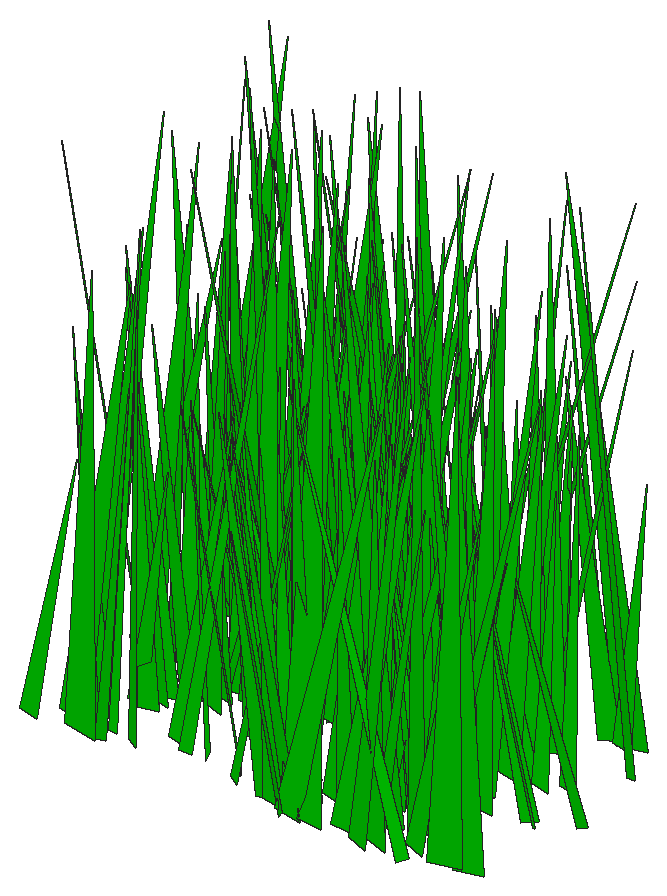
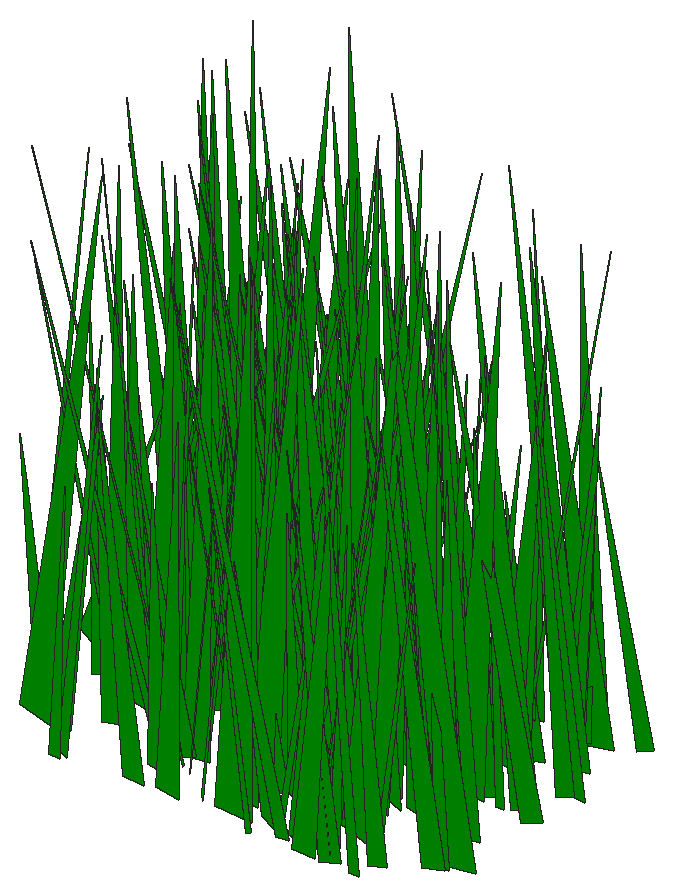
# SketchUp Ruby script. Lengths in inches.
U = 1.inch
M = Sketchup.active_model
def pt(a) = Geom::Point3d.new(a.map { |v| v * U })
def face(e, loops, mat)
  f = e.add_face(loops[0].map { |a| pt(a) })
  loops[1..].each { |l| e.add_face(l.map { |a| pt(a) }).erase! }
  f.material = f.back_material = mat if mat
  f
end
# faces: each face lists its corners as indices into pts; further lists are holes
def faces(e, pts, list, mat = nil) = list.each { |f| face(e, (f[0].is_a?(Array) ? f : [f]).map { |l| l.map { |i| pts[i] } }, mat) }
# xy, xz, yz: faces in a plane at the given z, y or x. An outline is a flat list of corners, or four numbers for a rectangle; further outlines are holes
def ring(l) = l.size == 4 ? [[l[0], l[1]], [l[2], l[1]], [l[2], l[3]], [l[0], l[3]]] : l.each_slice(2).to_a
def flat(e, list, mat, &to3) = list.each { |f| face(e, (f[0].is_a?(Array) ? f : [f]).map { |l| ring(l).map { |u, v| to3.(u, v) } }, mat) }
def xy(e, z, list, mat = nil) = flat(e, list, mat) { |x, y| [x, y, z] }
def xz(e, y, list, mat = nil) = flat(e, list, mat) { |x, z| [x, y, z] }
def yz(e, x, list, mat = nil) = flat(e, list, mat) { |y, z| [x, y, z] }
def lines(e, pts, list) = list.each { |a, b| e.add_line(pt(pts[a]), pt(pts[b])) }
# prism: a flat outline (further loops are holes) pulled along v
def prism(e, loops, v, mat = nil)
  f = face(e, loops, mat); d = Geom::Vector3d.new(v.map { |x| x * U })
  f.pushpull(f.normal.samedirection?(d) ? d.length : -d.length)
end
def box(e, o, s, mat = nil) = prism(e, [[o, [o[0] + s[0], o[1], o[2]], [o[0] + s[0], o[1] + s[1], o[2]], [o[0], o[1] + s[1], o[2]]]], [0, 0, s[2]], mat)
def at(x, y, z, deg = 0) = Geom::Transformation.translation(pt([x, y, z])) * Geom::Transformation.rotation(ORIGIN, Z_AXIS, deg.degrees)
def axes(o, x, y, z) = Geom::Transformation.new([*x, 0, *y, 0, *z, 0, *pt(o).to_a, 1])
def part(name) = M.definitions.add(name)
# library, detail: a bought-in or finely detailed component or shape, given as its bounding box
def library(name, o, s) = part(name).tap { |d| box(d.entities, o, s) }
def detail(e, o, s) = box(e.add_group.entities, o, s)
def put(e, d, t, mat = nil) = e.add_instance(d, t).tap { |i| i.material = mat if mat }
def group(e, t, mat = nil) = e.add_group.tap { |g| g.transformation = t; g.material = mat if mat }.entities
root = M.entities
M.materials.add("[Color G06]").color = [0, 204, 0]
c1 = part("fur_instance\#9")
p = [[0.8125,0,1.79],[0.67,-0.02,1.48],[0,-0.11,0],[0,0.11,0]]
faces(c1.entities,p,[[0,1,2,3]])
put(root,c1,axes([40.53,23.96,4.28],[1.83566,-0.31404,0.82516],[-2.24652,-0.26519,-0.43024],[-0.57423,0.03357,4.32098]),"[Color G06]")
put(root,c1,axes([40.32,19.16,4.28],[2.925,-0.2994,2.00765],[-2.40026,-0.41902,0.63304],[-0.80821,0.16086,5.38591]),"[Color G06]")
put(root,c1,axes([40.86,23.3,4.28],[-0.50928,-0.53289,0.41189],[-3.81061,0.07448,0.545],[0.39862,0.03119,5.73614]),"[Color G06]")
put(root,c1,axes([42.43,18.3,4.28],[-5.4088,-0.14631,1.26434],[-1.01838,0.76324,0.41425],[0.88283,-0.01595,8.22411]),"[Color G06]")
put(root,c1,axes([40.21,16.03,4.28],[1.67962,-0.32163,0.71269],[-2.35028,-0.22356,0.78271],[0.15328,0.09642,4.19195]),"[Color G06]")
put(root,c1,axes([41.55,17.18,4.28],[-3.0174,-0.25326,2.13427],[-2.1423,0.42935,-0.91281],[0.86507,0.17987,5.18387]),"[Color G06]")
put(root,c1,axes([40.09,23.79,4.28],[2.65212,0.74047,1.66794],[5.42605,-0.36092,-0.86575],[0.03104,-0.17528,8.82884]),"[Color G06]")
put(root,c1,axes([41.8,17.05,4.28],[-0.48262,0.51036,0.65675],[3.66206,0.05931,0.71626],[-0.42152,-0.06903,5.47073]),"[Color G06]")
put(root,c1,axes([40.62,22.84,4.28],[5.30556,0.09639,2.6107],[0.88862,-0.77174,-0.76063],[-1.65512,-0.10536,7.96032]),"[Color G06]")
put(root,c1,axes([40.95,22.4375,4.28],[1.49761,0.59441,2.65915],[4.61171,-0.20715,-0.48249],[-0.2609,-0.24951,6.73537]),"[Color G06]")
put(root,c1,axes([40.2,19.02,4.28],[5.10251,-0.47895,1.27674],[-3.39615,-0.7214,-0.76953],[-0.99644,0.00615,9.16059]),"[Color G06]")
put(root,c1,axes([42.05,24.64,4.28],[-2.97635,-0.1182,1.25222],[-1.01929,0.41533,-0.90804],[0.61772,0.11579,4.53526]),"[Color G06]")
put(root,c1,axes([40.82,23.28,4.28],[1.33282,-0.44936,2.42303],[-3.6069,-0.16234,0.97326],[0.05488,0.24351,5.12025]),"[Color G06]")
put(root,c1,axes([40.58,24.19,4.28],[2.21061,0.4766,1.81897],[3.62785,-0.29262,-1.04094],[-0.04082,-0.19545,5.99386]),"[Color G06]")
put(root,c1,axes([40.64,20.39,4.28],[-3.06048,0.47433,4.33015],[3.79536,0.53439,-0.73256],[2.35796,-0.2445,6.7994]),"[Color G06]")
put(root,c1,axes([41.25,20.64,4.28],[3.83688,0.20229,2.51337],[1.68851,-0.56978,-0.4898],[-1.4427,-0.12887,6.11109]),"[Color G06]")
put(root,c1,axes([40.14,20.73,4.28],[3.62063,-0.40355,0.80056],[-2.94205,-0.49947,0.79896],[-0.07963,0.10494,6.88125]),"[Color G06]")
put(root,c1,axes([41.74,16.69,4.28],[-1.39632,-0.40039,0.44175],[-2.8352,0.19884,0.68448],[0.54155,0.00863,4.72252]),"[Color G06]")
put(root,c1,axes([42.38,20.6,4.28],[-2.24292,0.64496,2.11415],[4.82593,0.31288,0.47182],[0.32145,-0.19707,7.66805]),"[Color G06]")
put(root,c1,axes([42.47,18.85,4.28],[-2.28583,0.50074,1.86531],[3.79192,0.31483,0.67108],[0.27173,-0.18103,6.32651]),"[Color G06]")
put(root,c1,axes([42.39,19.83,4.28],[-2.29137,-0.34724,1.45813],[-2.64251,0.32156,-0.47899],[0.4122,0.13116,5.03487]),"[Color G06]")
put(root,c1,axes([41.04,17.93,4.28],[2.09259,-0.65174,1.03361],[-4.7247,-0.28889,0.4409],[-0.01045,0.10483,7.64084]),"[Color G06]")
put(root,c1,axes([41.93,20.44,4.28],[-1.85847,0.47642,0.8115],[3.34872,0.26932,-1.03239],[0.868,-0.01898,5.72039]),"[Color G06]")
put(root,c1,axes([42.33,18.61,4.28],[-2.14148,-0.56177,0.67444],[-4.00795,0.30408,0.66903],[0.60798,0.02585,6.78597]),"[Color G06]")
put(root,c1,axes([41.24,16.61,4.28],[1.28342,0.62323,1.17804],[4.52586,-0.1673,-0.84654],[0.33624,-0.12697,6.89799]),"[Color G06]")
put(root,c1,axes([41.84,16.08,4.28],[-1.11415,-0.62905,1.94244],[-4.61886,0.18021,0.78614],[0.83987,0.15655,6.90014]),"[Color G06]")
put(root,c1,axes([42.48,18.11,4.28],[0.22403,0.44787,0.86974],[3.2356,-0.0412,0.5755],[-0.43055,-0.07657,4.77743]),"[Color G06]")
put(root,c1,axes([41.62,22.88,4.28],[3.59236,0.05386,1.44886],[0.30458,-0.51761,0.52335],[-0.99807,0.03588,5.37457]),"[Color G06]")
put(root,c1,axes([41.79,24.97,4.28],[-0.8526,-0.38753,1.77464],[-2.89615,0.15392,0.75311],[0.86337,0.13363,4.27882]),"[Color G06]")
put(root,c1,axes([43.27,24.02,4.28],[-4.05843,-0.54944,2.97754],[-4.30697,0.5757,-0.90957],[0.97164,0.25695,8.40497]),"[Color G06]")
put(root,c1,axes([42,25.67,4.28],[-4.01652,-0.27595,3.91009],[-2.0892,0.65983,0.5555],[2.52897,0.10683,6.66893]),"[Color G06]")
put(root,c1,axes([42.06,18.19,4.28],[0.69793,-0.37329,0.01251],[-2.65166,-0.09624,0.57094],[0.36756,0.01456,4.0951]),"[Color G06]")
put(root,c1,axes([42.77,22.1875,4.28],[2.46004,0.38232,1.76709],[2.81339,-0.36835,0.40627],[-0.99995,-0.09579,5.4904]),"[Color G06]")
put(root,c1,axes([42.49,16.63,4.28],[4.81574,-0.06122,2.66115],[-0.61978,-0.71096,0.62647],[-1.72596,0.08449,7.20012]),"[Color G06]")
put(root,c1,axes([42.52,16.09,4.28],[2.99416,0.27789,1.2227],[1.94849,-0.43266,0.63778],[-0.9187,-0.01196,5.33758]),"[Color G06]")
put(root,c1,axes([43.8,22.57,4.28],[-3.84297,-0.58383,2.53973],[-4.44087,0.54543,-0.60663],[0.83405,0.21407,8.47214]),"[Color G06]")
put(root,c1,axes([43.69,25.62,4.28],[-3.46173,0.39015,2.13045],[3.01439,0.49577,0.51133],[0.87953,-0.16354,6.63273]),"[Color G06]")
put(root,c1,axes([43.21,24.95,4.28],[-2.53132,-0.28053,1.18798],[-1.90201,0.36992,0.98175],[1.03016,-0.00632,4.73173]),"[Color G06]")
put(root,c1,axes([43.27,16.46,4.28],[3.80783,0.17226,2.69733],[1.4721,-0.57557,-0.41947],[-1.61744,-0.1183,5.96835]),"[Color G06]")
put(root,c1,axes([42.86,25.58,4.28],[-0.33449,-0.43562,1.904],[-3.28119,0.08352,0.90756],[0.78461,0.16358,4.60708]),"[Color G06]")
put(root,c1,axes([43.67,19.73,4.28],[-2.67306,-0.38143,1.59729],[-2.77779,0.39379,0.41882],[0.95304,0.07794,5.70076]),"[Color G06]")
put(root,c1,axes([43.68,20.45,4.28],[3.54777,0.50716,3.16085],[3.77954,-0.55366,0.72889],[-1.84809,-0.15869,7.55853]),"[Color G06]")
put(root,c1,axes([43.63,20.8,4.28],[3.54665,-0.38548,2.61839],[-2.74139,-0.54668,-0.95108],[-1.78772,0.07356,6.65306]),"[Color G06]")
put(root,c1,axes([43.7,21.86,4.28],[-2.08007,-0.31831,1.20851],[-2.30112,0.30611,0.41481],[0.75448,0.05606,4.59692]),"[Color G06]")
put(root,c1,axes([42.88,25.46,4.28],[3.86973,0.00845,1.35062],[0.16874,-0.55,-0.68461],[-0.88986,-0.06754,5.74365]),"[Color G06]")
put(root,c1,axes([43.54,22.17,4.28],[2.21799,0.39946,0.97771],[2.81815,-0.32155,0.81109],[-0.83202,-0.02424,5.35367]),"[Color G06]")
put(root,c1,axes([44.09,25.21,4.28],[1.27172,-0.47636,1.64511],[-3.46247,-0.20571,-0.86364],[-0.94486,0.11266,5.37906]),"[Color G06]")
put(root,c1,axes([43.65,19.21,4.28],[-2.68653,-0.47369,2.69346],[-3.52133,0.42622,0.76526],[1.54506,0.14776,6.42744]),"[Color G06]")
put(root,c1,axes([44.64,23.59,4.28],[-3.49736,-0.11002,1.11611],[-0.68296,0.49567,0.83226],[0.8448,-0.05474,5.29338]),"[Color G06]")
put(root,c1,axes([45.33,22.74,4.28],[-5.42496,-0.13003,1.43497],[-0.89547,0.76804,0.43282],[0.99473,-0.01775,8.21551]),"[Color G06]")
put(root,c1,axes([45.33,24.4375,4.28],[-5.08578,-0.13234,1.50166],[-1.05563,0.71679,-0.72938],[0.89209,0.09373,7.69781]),"[Color G06]")
put(root,c1,axes([44,20.2,4.28],[1.53141,0.77236,1.54184],[5.60337,-0.22434,0.47772],[-0.58749,-0.12637,8.57548]),"[Color G06]")
put(root,c1,axes([45.8,22.41,4.28],[-4.37992,0.25585,0.0158],[1.82006,0.60633,-0.85959],[0.2319,0.07341,7.04501]),"[Color G06]")
put(root,c1,axes([44.92,20.38,4.28],[-4.32277,-0.5601,2.74153],[-4.13834,0.63874,0.41513],[1.54027,0.14421,8.80946]),"[Color G06]")
put(root,c1,axes([44.35,21.96,4.28],[0.53574,0.73252,2.59344],[5.53098,-0.06561,-0.42351],[0.12093,-0.2446,7.88054]),"[Color G06]")
put(root,c1,axes([43.88,20.75,4.28],[3.11506,0.09524,0.56652],[0.59965,-0.43083,0.9554],[-0.50062,0.07659,4.66955]),"[Color G06]")
put(root,c1,axes([43.46,20.08,4.28],[3.4494,-0.09986,0.01085],[-0.71347,-0.47963,-0.40057],[-0.06156,-0.03639,5.25004]),"[Color G06]")
put(root,c1,axes([43.76,23.38,4.28],[3.74413,-0.55992,2.02858],[-4.21726,-0.51738,0.98225],[-0.42385,0.20181,8.14635]),"[Color G06]")
put(root,c1,axes([45.85,20.84,4.28],[-3.90579,-0.50598,0.67451],[-3.57993,0.54791,0.90985],[0.7443,-0.01986,7.91571]),"[Color G06]")
put(root,c1,axes([45.23,17.125,4.28],[-3.38063,-0.02034,1.9412],[0.10688,0.49628,1.01313],[1.30262,-0.09351,4.95479]),"[Color G06]")
put(root,c1,axes([44.18,17.23,4.28],[-1.69191,0.34093,3.20338],[2.703,0.33473,-0.90342],[1.80695,-0.18151,4.35087]),"[Color G06]")
put(root,c1,axes([44.49,22.05,4.28],[3.04168,0.0061,0.88041],[-0.0205,-0.42953,0.50031],[-0.59034,0.04637,4.51888]),"[Color G06]")
put(root,c1,axes([44.92,23.5,4.28],[4.1184,0.52375,2.39494],[3.77779,-0.60916,0.79207],[-1.5502,-0.09307,8.29285]),"[Color G06]")
put(root,c1,axes([45.4375,18.66,4.28],[-2.74931,-0.34755,1.10427],[-2.40812,0.39698,0.96016],[0.97908,0.00048,5.46241]),"[Color G06]")
put(root,c1,axes([44.72,19.82,4.28],[-1.3001,0.73831,2.86025],[5.51508,0.22204,-0.98452],[1.13102,-0.23405,8.08856]),"[Color G06]")
put(root,c1,axes([46.69,18.23,4.28],[-3.45537,0.00324,0.0516],[0.02659,0.47943,0.51793],[0.03202,-0.04836,5.13839]),"[Color G06]")
put(root,c1,axes([46.43,16.98,4.28],[-3.57778,-0.05248,0.80427],[-0.32446,0.50266,0.54396],[0.57093,-0.04323,5.34918]),"[Color G06]")
put(root,c1,axes([45.09,20.72,4.28],[-0.26976,-0.48293,0.07495],[-3.41337,0.03826,0.87515],[0.58768,0.00053,5.11744]),"[Color G06]")
put(root,c1,axes([45.61,23.5,4.28],[1.1975,0.38095,0.59823],[2.71746,-0.17338,0.53228],[-0.48865,-0.03064,4.42613]),"[Color G06]")
put(root,c1,axes([45.86,21.41,4.28],[4.2339,0.38734,4.51987],[3.51089,-0.65561,-0.8921],[-2.12957,-0.31078,7.5154]),"[Color G06]")
put(root,c1,axes([47.5,18.43,4.28],[-5.50039,-0.35127,0.42615],[-2.48534,0.7659,0.86803],[0.50014,-0.05724,9.00011]),"[Color G06]")
put(root,c1,axes([44.16,20.48,4.28],[5.67814,-0.09776,1.11475],[-0.64205,-0.79672,-0.72143],[-0.79726,-0.05467,8.52035]),"[Color G06]")
put(root,c1,axes([45.41,24.92,4.28],[2.03465,0.28036,0.01806],[1.95762,-0.2768,0.95653],[-0.45822,0.06233,4.1667]),"[Color G06]")
put(root,c1,axes([44.62,22.39,4.28],[2.8738,0.31849,0.51615],[2.30946,-0.39461,-0.75167],[0.04649,-0.08483,5.43464]),"[Color G06]")
put(root,c1,axes([45.82,18.77,4.28],[1.6438,0.51477,0.17214],[3.62988,-0.22842,1.03929],[-0.68165,0.02501,5.94944]),"[Color G06]")
put(root,c1,axes([46.24,19.05,4.28],[-0.14117,0.42924,2.02551],[3.34975,0.00096,0.49816],[-0.30202,-0.19,4.57841]),"[Color G06]")
put(root,c1,axes([46.78,23.54,4.28],[-2.18138,0.70767,1.33575],[5.15274,0.30094,0.48156],[0.05247,-0.13228,8.24177]),"[Color G06]")
put(root,c1,axes([46.87,17.7,4.28],[-3.40677,0.09208,0.72673],[0.57182,0.47441,-0.91758],[0.5878,0.07217,5.10462]),"[Color G06]")
put(root,c1,axes([45.01,21.19,4.28],[4.80966,-0.13527,1.46186],[-0.88572,-0.68305,-0.75104],[-1.05507,-0.04322,7.29457]),"[Color G06]")
put(root,c1,axes([45.89,18.58,4.28],[-2.85787,0.65388,3.16478],[4.9396,0.4432,-0.55519],[1.43946,-0.22267,8.18847]),"[Color G06]")
put(root,c1,axes([47.61,23.42,4.28],[-3.39013,-0.22695,0.06966],[-1.62254,0.46967,-0.61068],[-0.13508,0.05416,5.58713]),"[Color G06]")
put(root,c1,axes([45.45,25.66,4.28],[3.08314,0.13568,1.22761],[1.08935,-0.43642,-0.5702],[-0.65935,-0.08658,4.79824]),"[Color G06]")
put(root,c1,axes([46.34,25.14,4.28],[1.51104,-0.69587,3.03177],[-5.30597,-0.24298,-0.49936],[-0.92978,0.25568,7.77675]),"[Color G06]")
put(root,c1,axes([44.54,22.41,4.28],[3.65847,0.36053,0.29643],[2.59111,-0.50642,-0.67775],[0.10083,-0.06757,6.66108]),"[Color G06]")
put(root,c1,axes([44.65,16.9375,4.28],[5.79013,-0.15895,1.50969],[-1.22517,-0.81503,0.63879],[-0.90473,0.08646,8.7967]),"[Color G06]")
put(root,c1,axes([44.58,25.35,4.28],[4.61689,0.34082,0.70391],[2.4803,-0.64154,-0.65645],[-0.20845,-0.08497,7.77987]),"[Color G06]")
put(root,c1,axes([45.83,19.88,4.28],[3.33308,0.36634,1.18691],[2.61953,-0.47661,0.46723],[-0.81888,-0.03353,6.32569]),"[Color G06]")
put(root,c1,axes([46.59,24.4,4.28],[-3.60093,0.40203,3.79232],[3.51508,0.54041,0.87437],[1.54745,-0.29204,6.83862]),"[Color G06]")
put(root,c1,axes([47.15,23.74,4.28],[-4.03491,0.16334,2.0403],[1.33003,0.58567,0.48929],[1.21106,-0.09901,6.26034]),"[Color G06]")
put(root,c1,axes([45.81,21.72,4.28],[3.29128,-0.41256,1.812],[-3.13796,-0.46334,0.61316],[-0.61339,0.15665,6.58587]),"[Color G06]")
put(root,c1,axes([47.72,20.08,4.28],[-5.57827,-0.29111,2.54569],[-2.33628,0.79464,-0.99663],[1.34211,0.17331,8.84589]),"[Color G06]")
put(root,c1,axes([46.96,19.16,4.28],[1.23435,0.45739,1.78271],[3.37383,-0.20155,0.72226],[-0.89386,-0.12911,5.18792]),"[Color G06]")
put(root,c1,axes([48.52,22.58,4.28],[-4.50899,-0.39483,0.64193],[-2.86383,0.62197,-0.98755],[0.0084,0.10989,7.89603]),"[Color G06]")
put(root,c1,axes([46.89,20.58,4.28],[1.30755,0.44176,1.29397],[3.18621,-0.20213,0.73538],[-0.796,-0.08344,5.06913]),"[Color G06]")
put(root,c1,axes([46.82,23.08,4.28],[-4.51852,-0.39906,4.10548],[-3.45179,0.68164,-0.87497],[1.95457,0.28125,7.94572]),"[Color G06]")
put(root,c1,axes([47.25,17.13,4.28],[-3.04626,0.24969,1.73252],[1.95485,0.43956,0.40067],[0.8535,-0.11559,5.2659]),"[Color G06]")
put(root,c1,axes([48.27,17.78,4.28],[-3.22572,0.18767,0.14058],[1.34462,0.44445,0.76012],[-0.11002,-0.07047,5.16826]),"[Color G06]")
put(root,c1,axes([47.52,24.95,4.28],[-3.75893,-0.0662,1.61492],[-0.60194,0.54019,-0.5858],[1.01518,0.07517,5.63225]),"[Color G06]")
put(root,c1,axes([46.13,23.54,4.28],[2.29669,0.39301,1.40729],[2.97135,-0.30528,-1.03837],[-0.02751,-0.16313,5.3336]),"[Color G06]")
put(root,c1,axes([46.75,22.47,4.28],[3.20771,-0.21455,2.03857],[-1.7355,-0.47152,0.39925],[-1.10262,0.118,5.30211]),"[Color G06]")
put(root,c1,axes([47.85,16.36,4.28],[-0.93985,-0.54955,0.35892],[-3.93485,0.12753,-0.5846],[-0.3257,0.0451,6.027]),"[Color G06]")
put(root,c1,axes([44.97,22.71,4.28],[5.79154,0.20904,0.41951],[1.51707,-0.80538,-0.6829],[-0.15632,-0.07153,8.91502]),"[Color G06]")
put(root,c1,axes([46.8,19.55,4.28],[2.41853,0.32724,0.33072],[2.29006,-0.33668,0.86057],[-0.55831,0.03658,4.96255]),"[Color G06]")
put(root,c1,axes([47.4375,17.62,4.28],[1.72135,-0.3685,1.6676],[-2.7233,-0.26694,-0.49678],[-0.90103,0.10281,4.6873]),"[Color G06]")
put(root,c1,axes([47.85,21.63,4.28],[1.99894,-0.65899,2.69846],[-4.88099,-0.3224,-0.96791],[-1.33004,0.19273,7.6076]),"[Color G06]")
put(root,c1,axes([46.91,20.45,4.28],[0.83169,-0.65828,1.18178],[-4.77084,-0.10498,0.7825],[0.38622,0.12078,7.1212]),"[Color G06]")
put(root,c1,axes([47.07,18.67,4.28],[2.76158,0.67742,2.84297],[5.17952,-0.39195,-0.50999],[-0.62494,-0.25501,8.33611]),"[Color G06]")
put(root,c1,axes([46.53,16.58,4.28],[3.46289,0.17722,0.73587],[1.32426,-0.48184,-0.58951],[-0.32246,-0.07561,5.48149]),"[Color G06]")
put(root,c1,axes([48.59,15.92,4.28],[-2.68808,-0.08471,0.62131],[-0.68917,0.36674,-0.91642],[0.25864,0.0968,4.01561]),"[Color G06]")
put(root,c1,axes([46.87,24.125,4.28],[3.39465,-0.03544,0.64985],[-0.16669,-0.46893,-0.9927],[-0.47525,-0.08867,4.98997]),"[Color G06]")
put(root,c1,axes([46.56,20.74,4.28],[3.53442,-0.02635,0.11084],[-0.17831,-0.48918,-0.66038],[-0.09707,-0.06099,5.24861]),"[Color G06]")
put(root,c1,axes([48.86,16.07,4.28],[-3.05052,-0.35844,0.15026],[-2.53255,0.42228,0.86964],[0.45112,-0.05313,5.89824]),"[Color G06]")
put(root,c1,axes([48.14,16.24,4.28],[-1.12886,-0.51523,0.36614],[-3.68038,0.16005,0.52596],[0.40852,0.01817,5.75024]),"[Color G06]")
put(root,c1,axes([48.65,24.02,4.28],[-2.84807,-0.0062,1.21061],[-0.19682,0.40529,-0.79568],[0.78699,0.07891,4.18215]),"[Color G06]")
put(root,c1,axes([48.34,25.34,4.28],[1.78389,-0.43619,1.55467],[-3.16698,-0.27255,-0.66714],[-0.91494,0.09293,5.34043]),"[Color G06]")
put(root,c1,axes([46.5625,20.57,4.28],[4.37368,-0.14503,0.02248],[-1.03587,-0.60814,-0.515],[-0.09431,-0.04626,6.6993]),"[Color G06]")
put(root,c1,axes([49.1,22.79,4.28],[-4.43003,-0.22421,1.48246],[-1.52848,0.6326,0.78811],[1.11037,-0.02374,6.9994]),"[Color G06]")
put(root,c1,axes([48.66,21.03,4.28],[1.15822,-0.38821,1.56672],[-2.84543,-0.19033,-0.71901],[-0.86775,0.10595,4.44887]),"[Color G06]")
put(root,c1,axes([47.43,20.84,4.28],[2.34909,-0.53687,1.3979],[-3.96198,-0.318,0.84274],[0.00824,0.15229,6.68775]),"[Color G06]")
put(root,c1,axes([48.67,16.9,4.28],[2.38709,-0.57744,2.75855],[-4.34986,-0.3737,-0.57808],[-1.27797,0.19337,7.12026]),"[Color G06]")
put(root,c1,axes([48.57,21.92,4.28],[-2.49341,0.09457,1.78886],[0.89911,0.37352,0.53102],[1.04121,-0.09608,3.82529]),"[Color G06]")
put(root,c1,axes([49.37,19.125,4.28],[-1.12072,-0.35899,0.25382],[-2.56971,0.15302,-0.48397],[-0.23012,0.03963,4.16841]),"[Color G06]")
put(root,c1,axes([48.9,23.48,4.28],[-2.90028,-0.61954,1.92635],[-4.47596,0.42941,0.81185],[1.16894,0.1071,7.88817]),"[Color G06]")
put(root,c1,axes([49.26,18.79,4.28],[-1.07389,0.47209,2.07133],[3.6582,0.13812,0.62028],[-0.00848,-0.20173,5.272]),"[Color G06]")
put(root,c1,axes([48.91,20.55,4.28],[1.9479,0.43829,1.73229],[3.2045,-0.29828,0.62058],[-0.97658,-0.10455,5.49162]),"[Color G06]")
put(root,c1,axes([48.42,19.92,4.28],[3.72685,-0.30006,1.57967],[-2.12855,-0.5395,-0.55487],[-1.10306,0.02726,6.40786]),"[Color G06]")
put(root,c1,axes([47.75,21.86,4.28],[5.67179,-0.23551,1.61942],[-1.62764,-0.80491,-0.71325],[-1.17354,-0.02186,8.81594]),"[Color G06]")
put(root,c1,axes([49.61,18.32,4.28],[-0.84016,-0.72392,0.69324],[-5.20529,0.1132,-0.51251],[-0.26588,0.07138,7.84315]),"[Color G06]")
put(root,c1,axes([49.16,16.22,4.28],[-1.90552,-0.58279,1.04932],[-4.15603,0.27798,0.8769],[0.82893,0.05402,6.80869]),"[Color G06]")
put(root,c1,axes([49.9,19.91,4.28],[-4.61908,-0.3088,1.96866],[-2.18599,0.66925,0.60225],[1.36395,0.02684,7.6322]),"[Color G06]")
put(root,c1,axes([49.3,24.55,4.28],[0.63735,0.42213,0.33956],[3.01795,-0.09161,0.42904],[-0.32827,-0.0226,4.60366]),"[Color G06]")
put(root,c1,axes([47.99,20.86,4.28],[3.19918,0.49675,0.80907],[3.60232,-0.43872,-0.87487],[0.0793,-0.11063,7.1023]),"[Color G06]")
put(root,c1,axes([48.02,22.02,4.28],[4.52651,-0.07013,0.83094],[-0.57359,-0.62949,0.87636],[-0.48274,0.09036,6.75019]),"[Color G06]")
put(root,c1,axes([49.7,19.15,4.28],[0.34802,-0.46943,1.5699],[-3.5035,-0.06281,-0.42272],[-0.40222,0.14094,5.04052]),"[Color G06]")
put(root,c1,axes([49.34,23.12,4.28],[2.50264,0.14898,1.8484],[1.32653,-0.3694,-0.59168],[-0.9546,-0.12276,4.02367]),"[Color G06]")
put(root,c1,axes([49.16,16.02,4.28],[-0.04869,0.77204,3.65771],[6.03843,0.03008,-0.54985],[0.42369,-0.34001,8.25673]),"[Color G06]")
put(root,c1,axes([49.69,17.23,4.28],[-1.96551,-0.41978,1.13769],[-2.97553,0.29054,0.83201],[0.8876,0.04443,5.30847]),"[Color G06]")
put(root,c1,axes([50.15,21.25,4.28],[-1.88157,0.36031,0.04215],[2.55123,0.25981,-0.72804],[0.4102,0.03685,4.72135]),"[Color G06]")
put(root,c1,axes([49.08,21.27,4.28],[0.94242,0.57195,0.95476],[4.13273,-0.12071,-0.80548],[0.38939,-0.10313,6.23807]),"[Color G06]")
put(root,c1,axes([50.28,18.47,4.28],[-4.21447,0.31774,2.85755],[2.59286,0.61902,0.63499],[1.45768,-0.18242,7.13233]),"[Color G06]")
put(root,c1,axes([49.79,19.83,4.28],[-1.04988,0.34218,0.66756],[2.42438,0.15588,-0.66164],[0.58593,-0.03185,3.9338]),"[Color G06]")
put(root,c1,axes([49.08,23.53,4.28],[2.44901,0.28457,0.85121],[2.11835,-0.3311,-0.89843],[-0.03878,-0.11535,4.67895]),"[Color G06]")
put(root,c1,axes([50.02,18.33,4.28],[-1.50955,0.32927,0.89223],[2.31511,0.22441,-0.76414],[0.75659,-0.0297,4.11839]),"[Color G06]")
put(root,c1,axes([50.43,22.41,4.28],[-4.3213,-0.15313,2.62349],[-1.32076,0.64012,-0.56739],[1.5946,0.11521,6.63958]),"[Color G06]")
put(root,c1,axes([49.29,17.33,4.28],[2.31989,0.5755,1.7522],[4.2881,-0.31705,-0.71933],[-0.13927,-0.17565,7.03927]),"[Color G06]")
put(root,c1,axes([49.43,25.37,4.28],[2.5056,-0.39652,0.1136],[-2.8262,-0.34862,-0.54278],[-0.32255,-0.02557,5.63829]),"[Color G06]")
put(root,c1,axes([51.04,19.71,4.28],[-4.45941,0.33978,2.36404],[2.64631,0.64184,0.5532],[1.19848,-0.15292,7.57481]),"[Color G06]")
put(root,c1,axes([51.15,17.18,4.28],[-3.32144,-0.62591,2.81548],[-4.82527,0.4653,-0.83271],[0.64229,0.25888,8.30378]),"[Color G06]")
put(root,c1,axes([48.76,15.99,4.28],[3.34696,-0.48122,0.42602],[-3.45002,-0.4587,1.02415],[0.29634,0.09488,7.11169]),"[Color G06]")
put(root,c1,axes([52.5625,15.97,4.28],[-4.4445,0.21407,0.10298],[1.53376,0.61616,0.72958],[-0.09461,-0.06747,6.98973]),"[Color G06]")
put(root,c1,axes([51.42,18.05,4.28],[-2.49171,0.37221,1.25779],[2.77587,0.34872,0.42896],[0.35719,-0.11355,5.44054]),"[Color G06]")
put(root,c1,axes([50.81,19.29,4.28],[-2.1954,-0.41957,1.99156],[-3.11509,0.33698,0.48472],[1.0607,0.12122,5.54561]),"[Color G06]")
put(root,c1,axes([50.57,18.08,4.28],[-1.44883,0.41297,2.77466],[3.29087,0.2556,-0.53164],[1.17778,-0.20617,4.89869]),"[Color G06]")
put(root,c1,axes([51.94,17.625,4.28],[-4.25672,0.08608,1.50094],[0.69903,0.60683,0.43055],[0.94917,-0.06088,6.41409]),"[Color G06]")
put(root,c1,axes([50.13,18.63,4.28],[3.25581,0.08594,0.49881],[0.55815,-0.45168,0.8021],[-0.42392,0.06536,4.88708]),"[Color G06]")
put(root,c1,axes([50.52,21.54,4.28],[-0.44097,-0.69185,2.91082],[-5.26513,0.09893,0.91942],[0.82904,0.26029,7.38745]),"[Color G06]")
put(root,c1,axes([51.73,25.39,4.28],[-3.905,-0.20913,1.8696],[-1.64828,0.56209,-0.46746],[1.04745,0.10486,6.23443]),"[Color G06]")
put(root,c1,axes([52.35,19.93,4.28],[-2.94823,0.02639,0.06701],[0.19376,0.40679,0.63789],[0.01693,-0.0598,4.3691]),"[Color G06]")
put(root,c1,axes([51.76,17.8125,4.28],[0.18514,-0.49731,0.34422],[-3.50617,-0.0315,-1.01546],[-0.69165,0.02656,5.2398]),"[Color G06]")
put(root,c1,axes([50.72,16.6,4.28],[3.39782,-0.32776,1.34076],[-2.33017,-0.48926,-0.54849],[-0.9485,0.02782,6.15051]),"[Color G06]")
put(root,c1,axes([50.73,18.76,4.28],[0.47502,-0.8177,1.78012],[-5.96414,-0.05125,0.85084],[0.48322,0.17131,8.75154]),"[Color G06]")
put(root,c1,axes([51.1,20.24,4.28],[1.97954,-0.5012,0.13626],[-3.54315,-0.27441,-0.96744],[-0.61057,-0.03256,6.05588]),"[Color G06]")
put(root,c1,axes([50.55,22.98,4.28],[5.21535,0.22618,2.03704],[1.5611,-0.75167,0.65951],[-1.43228,0.0043,8.1363]),"[Color G06]")
put(root,c1,axes([52.63,21.2,4.28],[-2.79097,0.31278,0.32413],[2.2504,0.38435,0.67881],[-0.11736,-0.06825,5.30821]),"[Color G06]")
put(root,c1,axes([48.91,23.99,4.28],[6.07479,0.10569,0.0761],[0.75938,-0.84328,-0.86223],[0.02113,-0.08071,9.1089]),"[Color G06]")
put(root,c1,axes([51.67,21.64,4.28],[-2.4328,0.45129,3.20878],[3.79115,0.35262,0.72342],[0.84287,-0.2835,6.00774]),"[Color G06]")
put(root,c1,axes([52.66,18.7,4.28],[-3.51601,-0.03478,0.45972],[-0.29598,0.48541,-0.83769],[0.2631,0.08125,5.20112]),"[Color G06]")
put(root,c1,axes([49.4375,24.17,4.28],[5.18964,-0.0143,0.01698],[-0.10315,-0.71992,0.7891],[-0.00087,0.07364,7.71757]),"[Color G06]")
put(root,c1,axes([52.1875,19.63,4.28],[-2.8516,0.11009,1.16694],[0.93363,0.40015,0.75964],[0.60103,-0.09926,4.35651]),"[Color G06]")
put(root,c1,axes([51.42,16.21,4.28],[-1.7675,-0.49886,1.25927],[-3.54502,0.26581,0.9818],[0.97006,0.06243,5.88239]),"[Color G06]")
put(root,c1,axes([51.9375,21.22,4.28],[-1.76556,-0.31835,0.32018],[-2.25828,0.24795,0.50412],[0.39772,-0.00538,4.28386]),"[Color G06]")
put(root,c1,axes([51.8,25.63,4.28],[-2.19509,0.16349,1.65605],[1.38512,0.32476,0.41811],[0.8269,-0.11,3.69578]),"[Color G06]")
put(root,c1,axes([51.03,16.95,4.28],[2.79353,0.25757,1.25741],[1.98233,-0.38909,-0.68165],[-0.43588,-0.1188,4.95864]),"[Color G06]")
put(root,c1,axes([51.95,22.15,4.28],[1.00057,0.64288,0.38068],[4.57352,-0.14298,0.887],[-0.63442,-0.01686,6.9948]),"[Color G06]")
put(root,c1,axes([50.41,16.3,4.28],[3.53367,-0.50705,0.77867],[-3.67325,-0.48851,0.69304],[-0.02728,0.09718,7.54632]),"[Color G06]")
put(root,c1,axes([51.09,15.95,4.28],[4.15502,0.37853,2.105],[2.91508,-0.59039,-0.65706],[-0.92452,-0.16034,7.38865]),"[Color G06]")
put(root,c1,axes([52.78,24.21,4.28],[-1.35214,0.4491,1.14004],[3.30116,0.17473,0.83888],[-0.23828,-0.12781,5.15266]),"[Color G06]")
put(root,c1,axes([50.48,17.75,4.28],[4.17516,0.32489,0.63701],[2.36464,-0.57868,-0.71531],[-0.13617,-0.08733,7.11003]),"[Color G06]")
put(root,c1,axes([52.06,22.79,4.28],[-3.78756,0.40993,3.78743],[3.47719,0.57775,0.58399],[1.72424,-0.26463,7.14198]),"[Color G06]")
put(root,c1,axes([51.73,23.37,4.28],[-0.62528,-0.43903,1.11483],[-3.16905,0.10447,0.75584],[0.65274,0.08665,4.73753]),"[Color G06]")
put(root,c1,axes([52.07,19.87,4.28],[2.14117,0.42814,1.08708],[3.00305,-0.31413,0.99962],[-0.96823,-0.02751,5.50442]),"[Color G06]")
put(root,c1,axes([51.93,22.93,4.28],[-1.16581,0.48569,0.54852],[3.42534,0.16936,-0.96501],[0.73001,-0.01905,5.40396]),"[Color G06]")
put(root,c1,axes([52.18,17.02,4.28],[-4.74027,-0.36233,4.06824],[-3.12551,0.71907,-0.7779],[2.09573,0.25286,8.0417]),"[Color G06]")
put(root,c1,axes([52.57,17.81,4.28],[-0.14213,0.42821,0.9977],[3.12583,0.00966,0.51835],[-0.32386,-0.09468,4.56518]),"[Color G06]")
put(root,c1,axes([52.07,21.78,4.28],[-1.83498,0.43351,1.97418],[3.22133,0.28766,-0.56798],[1.01619,-0.12906,5.3654]),"[Color G06]")
put(root,c1,axes([51.43,21.85,4.28],[2.94578,0.46509,1.53896],[3.47279,-0.40945,-0.63387],[-0.35226,-0.14732,6.62044]),"[Color G06]")
put(root,c1,axes([51.49,19.3,4.28],[2.8531,-0.01386,0.26168],[-0.06202,-0.3905,-0.86464],[-0.19152,-0.07994,4.17823]),"[Color G06]")
put(root,c1,axes([51.85,21.14,4.28],[0.99967,-0.49246,2.19004],[-3.81513,-0.11452,0.93186],[0.25266,0.21925,5.40583]),"[Color G06]")
put(root,c1,axes([53.52,24.24,4.28],[-2.89657,-0.65517,2.10303],[-4.90159,0.39462,-0.95774],[0.17052,0.21429,8.1935]),"[Color G06]")
put(root,c1,axes([51.8125,18.69,4.28],[2.66664,0.19143,0.06493],[1.34994,-0.36773,0.7025],[-0.25331,0.05554,4.42722]),"[Color G06]")
put(root,c1,axes([52.3125,19.33,4.28],[0.14843,0.55941,3.68822],[4.6982,0.00667,-0.53859],[0.33184,-0.34467,5.9756]),"[Color G06]")
put(root,c1,axes([52.55,18.32,4.28],[-0.71319,-0.74708,2.79243],[-5.6494,0.1179,0.40041],[0.52722,0.25273,8.06789]),"[Color G06]")
put(root,c1,axes([54.13,19.42,4.28],[-3.78591,-0.00653,0.34322],[-0.06737,0.52672,-0.50839],[0.22448,0.04791,5.63587]),"[Color G06]")
put(root,c1,axes([53.86,19.61,4.28],[-1.6674,0.35264,0.25915],[2.50311,0.2245,0.88161],[-0.39965,-0.06515,4.44054]),"[Color G06]")
put(root,c1,axes([53.51,17.54,4.28],[-1.80478,-0.53249,1.60562],[-3.96433,0.248,-0.50564],[0.14196,0.15581,6.29227]),"[Color G06]")
put(root,c1,axes([53.01,18.06,4.28],[-2.86679,0.15539,1.63885],[0.98508,0.42754,-0.80751],[1.21396,0.02002,4.52544]),"[Color G06]")
put(root,c1,axes([51.78,22.85,4.28],[4.28076,0.24257,0.37594],[1.68939,-0.59333,1.0091],[-0.48509,0.07429,6.83188]),"[Color G06]")
put(root,c1,axes([52.44,17.44,4.28],[1.83499,-0.64887,1.71558],[-4.79242,-0.25036,0.57227],[-0.0544,0.16857,7.4539]),"[Color G06]")
put(root,c1,axes([52.94,21.17,4.28],[-1.87874,0.3065,1.49496],[2.16169,0.29223,-0.81436],[1.07654,-0.05189,4.24419]),"[Color G06]")
put(root,c1,axes([52.11,19.9,4.28],[4.70584,-0.3913,1.39358],[-2.80038,-0.66822,-0.43075],[-0.94947,0.03149,8.17739]),"[Color G06]")
put(root,c1,axes([52.43,16.61,4.28],[2.6321,0.36678,0.84421],[2.69022,-0.35928,-0.80456],[-0.01047,-0.1088,5.5029]),"[Color G06]")
put(root,c1,axes([54.48,22.99,4.28],[-5.10079,-0.24081,2.33991],[-1.88482,0.73514,-0.48669],[1.37146,0.11467,8.03385]),"[Color G06]")
put(root,c1,axes([53.29,24.12,4.28],[0.32029,0.36637,1.22399],[2.73791,-0.03078,-0.5419],[0.27858,-0.1187,3.91858]),"[Color G06]")
put(root,c1,axes([52.07,18.11,4.28],[4.2565,0.32543,0.62403],[2.36735,-0.58988,-0.73143],[-0.1281,-0.08791,7.21815]),"[Color G06]")
put(root,c1,axes([53.5625,21.54,4.28],[-2.54278,0.29753,2.06869],[2.17703,0.39574,-0.56102],[1.31492,-0.07983,4.92926]),"[Color G06]")
put(root,c1,axes([55.11,20.2,4.28],[-2.11196,-0.28159,0.10746],[-1.97418,0.28446,-1.04015],[-0.43063,0.07689,4.24145]),"[Color G06]")
put(root,c1,axes([54.28,16.55,4.28],[0.87323,0.66868,1.61696],[4.85745,-0.14092,0.83475],[-0.75541,-0.13315,7.23682]),"[Color G06]")
put(root,c1,axes([53.58,16.44,4.28],[2.10359,-0.6857,0.75588],[-4.91758,-0.29809,-0.49392],[-0.50373,0.04651,7.97833]),"[Color G06]")
